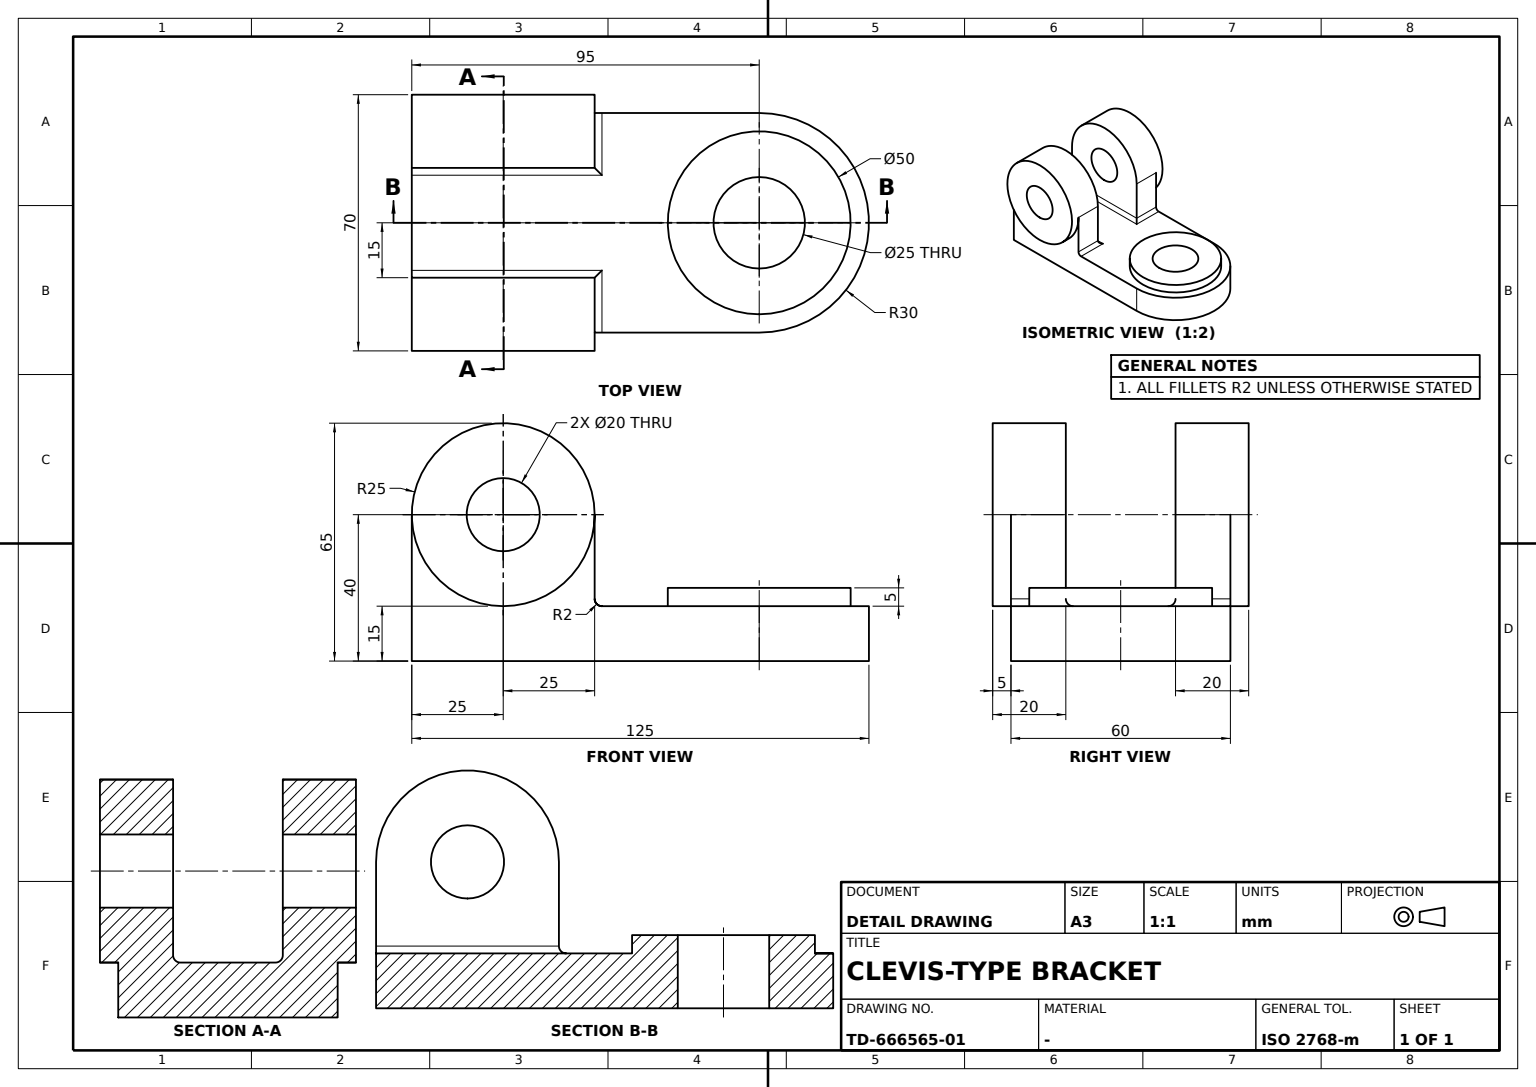
ISO-10303-21;
HEADER;
FILE_DESCRIPTION((''),'2;1');
FILE_NAME('','',(''),(''),'','','');
FILE_SCHEMA(('AUTOMOTIVE_DESIGN'));
ENDSEC;
DATA;
#1=APPLICATION_CONTEXT('');
#2=PRODUCT_CONTEXT('',#1,'mechanical');
#3=PRODUCT('','','',(#2));
#4=PRODUCT_DEFINITION_FORMATION('','',#3);
#5=PRODUCT_DEFINITION_CONTEXT('',#1,'design');
#6=PRODUCT_DEFINITION('','',#4,#5);
#7=PRODUCT_DEFINITION_SHAPE('','',#6);
#8=(LENGTH_UNIT()NAMED_UNIT(*)SI_UNIT(.MILLI.,.METRE.));
#9=(NAMED_UNIT(*)PLANE_ANGLE_UNIT()SI_UNIT($,.RADIAN.));
#10=(NAMED_UNIT(*)SI_UNIT($,.STERADIAN.)SOLID_ANGLE_UNIT());
#11=UNCERTAINTY_MEASURE_WITH_UNIT(LENGTH_MEASURE(0.005),#8,'distance_accuracy_value','');
#12=(GEOMETRIC_REPRESENTATION_CONTEXT(3)GLOBAL_UNCERTAINTY_ASSIGNED_CONTEXT((#11))GLOBAL_UNIT_ASSIGNED_CONTEXT((#8,#9,#10))REPRESENTATION_CONTEXT('',''));
#13=CARTESIAN_POINT('',(15.,-95.,40.));
#14=VERTEX_POINT('',#13);
#15=CARTESIAN_POINT('',(15.,-95.,17.));
#16=VERTEX_POINT('',#15);
#17=CARTESIAN_POINT('',(15.,-95.,0.));
#18=DIRECTION('',(0.,0.,-1.));
#19=VECTOR('',#18,1000.);
#20=LINE('',#17,#19);
#21=EDGE_CURVE('',#14,#16,#20,.T.);
#22=ORIENTED_EDGE('',*,*,#21,.F.);
#23=CARTESIAN_POINT('',(15.,-45.,40.));
#24=VERTEX_POINT('',#23);
#25=CARTESIAN_POINT('',(15.,-70.,40.));
#26=DIRECTION('',(1.,0.,0.));
#27=AXIS2_PLACEMENT_3D('',#25,#26,#18);
#28=CIRCLE('',#27,25.);
#29=EDGE_CURVE('',#24,#14,#28,.T.);
#30=ORIENTED_EDGE('',*,*,#29,.F.);
#31=CARTESIAN_POINT('',(15.,-45.,17.));
#32=VERTEX_POINT('',#31);
#33=CARTESIAN_POINT('',(15.,-45.,15.));
#34=DIRECTION('',(0.,0.,1.));
#35=VECTOR('',#34,1000.);
#36=LINE('',#33,#35);
#37=EDGE_CURVE('',#32,#24,#36,.T.);
#38=ORIENTED_EDGE('',*,*,#37,.F.);
#39=CARTESIAN_POINT('',(15.,-32.5,17.));
#40=DIRECTION('',(0.,1.,0.));
#41=VECTOR('',#40,1000.);
#42=LINE('',#39,#41);
#43=EDGE_CURVE('',#16,#32,#42,.T.);
#44=ORIENTED_EDGE('',*,*,#43,.F.);
#45=EDGE_LOOP('',(#22,#30,#38,#44));
#46=FACE_BOUND('',#45,.T.);
#47=CARTESIAN_POINT('',(15.,-70.,30.));
#48=VERTEX_POINT('',#47);
#49=CIRCLE('',#27,10.);
#50=EDGE_CURVE('',#48,#48,#49,.F.);
#51=ORIENTED_EDGE('',*,*,#50,.F.);
#52=EDGE_LOOP('',(#51));
#53=FACE_BOUND('',#52,.T.);
#54=CARTESIAN_POINT('',(15.,0.,0.));
#55=AXIS2_PLACEMENT_3D('',#54,#26,#40);
#56=PLANE('',#55);
#57=ADVANCED_FACE('',(#46,#53),#56,.F.);
#58=CARTESIAN_POINT('',(35.,-70.,30.));
#59=VERTEX_POINT('',#58);
#60=CARTESIAN_POINT('',(35.,-70.,40.));
#61=AXIS2_PLACEMENT_3D('',#60,#26,#18);
#62=CIRCLE('',#61,10.);
#63=EDGE_CURVE('',#59,#59,#62,.T.);
#64=ORIENTED_EDGE('',*,*,#63,.T.);
#65=EDGE_LOOP('',(#64));
#66=FACE_BOUND('',#65,.T.);
#67=ORIENTED_EDGE('',*,*,#50,.T.);
#68=EDGE_LOOP('',(#67));
#69=FACE_BOUND('',#68,.T.);
#70=CARTESIAN_POINT('',(-34.9,-70.,40.));
#71=AXIS2_PLACEMENT_3D('',#70,#26,#40);
#72=CYLINDRICAL_SURFACE('',#71,10.);
#73=ADVANCED_FACE('',(#66,#69),#72,.F.);
#74=CARTESIAN_POINT('',(30.,-95.,0.));
#75=VERTEX_POINT('',#74);
#76=CARTESIAN_POINT('',(30.,-95.,40.));
#77=VERTEX_POINT('',#76);
#78=LINE('',#74,#35);
#79=EDGE_CURVE('',#75,#77,#78,.T.);
#80=ORIENTED_EDGE('',*,*,#79,.F.);
#81=CARTESIAN_POINT('',(30.,0.,0.));
#82=VERTEX_POINT('',#81);
#83=LINE('',#81,#41);
#84=EDGE_CURVE('',#75,#82,#83,.T.);
#85=ORIENTED_EDGE('',*,*,#84,.T.);
#86=CARTESIAN_POINT('',(30.,0.,15.));
#87=VERTEX_POINT('',#86);
#88=CARTESIAN_POINT('',(30.,0.,7.5));
#89=LINE('',#88,#35);
#90=EDGE_CURVE('',#82,#87,#89,.T.);
#91=ORIENTED_EDGE('',*,*,#90,.T.);
#92=CARTESIAN_POINT('',(30.,-43.,15.));
#93=VERTEX_POINT('',#92);
#94=LINE('',#86,#41);
#95=EDGE_CURVE('',#93,#87,#94,.T.);
#96=ORIENTED_EDGE('',*,*,#95,.F.);
#97=CARTESIAN_POINT('',(30.,-45.,17.));
#98=VERTEX_POINT('',#97);
#99=CARTESIAN_POINT('',(30.,-43.,17.));
#100=AXIS2_PLACEMENT_3D('',#99,#26,#18);
#101=CIRCLE('',#100,2.);
#102=EDGE_CURVE('',#98,#93,#101,.T.);
#103=ORIENTED_EDGE('',*,*,#102,.F.);
#104=CARTESIAN_POINT('',(30.,-45.,40.));
#105=VERTEX_POINT('',#104);
#106=CARTESIAN_POINT('',(30.,-45.,15.));
#107=LINE('',#106,#35);
#108=EDGE_CURVE('',#98,#105,#107,.T.);
#109=ORIENTED_EDGE('',*,*,#108,.T.);
#110=CARTESIAN_POINT('',(30.,-70.,40.));
#111=AXIS2_PLACEMENT_3D('',#110,#26,#18);
#112=CIRCLE('',#111,25.);
#113=EDGE_CURVE('',#77,#105,#112,.T.);
#114=ORIENTED_EDGE('',*,*,#113,.F.);
#115=EDGE_LOOP('',(#80,#85,#91,#96,#103,#109,#114));
#116=FACE_BOUND('',#115,.T.);
#117=AXIS2_PLACEMENT_3D('',#74,#26,#40);
#118=PLANE('',#117);
#119=ADVANCED_FACE('',(#116),#118,.T.);
#120=CARTESIAN_POINT('',(25.,0.,15.));
#121=VERTEX_POINT('',#120);
#122=CARTESIAN_POINT('',(0.,0.,15.));
#123=AXIS2_PLACEMENT_3D('',#122,#34,#26);
#124=CIRCLE('',#123,25.);
#125=EDGE_CURVE('',#121,#121,#124,.T.);
#126=ORIENTED_EDGE('',*,*,#125,.F.);
#127=EDGE_LOOP('',(#126));
#128=FACE_BOUND('',#127,.T.);
#129=CARTESIAN_POINT('',(13.,-95.,15.));
#130=VERTEX_POINT('',#129);
#131=CARTESIAN_POINT('',(13.,-43.,15.));
#132=VERTEX_POINT('',#131);
#133=CARTESIAN_POINT('',(13.,-32.5,15.));
#134=LINE('',#133,#41);
#135=EDGE_CURVE('',#130,#132,#134,.T.);
#136=ORIENTED_EDGE('',*,*,#135,.T.);
#137=CARTESIAN_POINT('',(0.,-43.,15.));
#138=DIRECTION('',(-1.,0.,0.));
#139=VECTOR('',#138,1000.);
#140=LINE('',#137,#139);
#141=EDGE_CURVE('',#93,#132,#140,.T.);
#142=ORIENTED_EDGE('',*,*,#141,.F.);
#143=ORIENTED_EDGE('',*,*,#95,.T.);
#144=CARTESIAN_POINT('',(-30.,0.,15.));
#145=VERTEX_POINT('',#144);
#146=CIRCLE('',#123,30.);
#147=EDGE_CURVE('',#87,#145,#146,.T.);
#148=ORIENTED_EDGE('',*,*,#147,.T.);
#149=CARTESIAN_POINT('',(-30.,-43.,15.));
#150=VERTEX_POINT('',#149);
#151=DIRECTION('',(0.,-1.,0.));
#152=VECTOR('',#151,1000.);
#153=LINE('',#144,#152);
#154=EDGE_CURVE('',#145,#150,#153,.T.);
#155=ORIENTED_EDGE('',*,*,#154,.T.);
#156=CARTESIAN_POINT('',(-13.,-43.,15.));
#157=VERTEX_POINT('',#156);
#158=EDGE_CURVE('',#157,#150,#140,.T.);
#159=ORIENTED_EDGE('',*,*,#158,.F.);
#160=CARTESIAN_POINT('',(-13.,-95.,15.));
#161=VERTEX_POINT('',#160);
#162=CARTESIAN_POINT('',(-13.,-32.5,15.));
#163=LINE('',#162,#41);
#164=EDGE_CURVE('',#161,#157,#163,.T.);
#165=ORIENTED_EDGE('',*,*,#164,.F.);
#166=CARTESIAN_POINT('',(0.,-95.,15.));
#167=VECTOR('',#26,1000.);
#168=LINE('',#166,#167);
#169=EDGE_CURVE('',#161,#130,#168,.T.);
#170=ORIENTED_EDGE('',*,*,#169,.T.);
#171=EDGE_LOOP('',(#136,#142,#143,#148,#155,#159,#165,#170));
#172=FACE_BOUND('',#171,.T.);
#173=PLANE('',#123);
#174=ADVANCED_FACE('',(#128,#172),#173,.T.);
#175=CARTESIAN_POINT('',(32.5,-45.,40.));
#176=LINE('',#175,#167);
#177=EDGE_CURVE('',#105,#24,#176,.F.);
#178=ORIENTED_EDGE('',*,*,#177,.F.);
#179=ORIENTED_EDGE('',*,*,#108,.F.);
#180=CARTESIAN_POINT('',(0.,-45.,17.));
#181=LINE('',#180,#139);
#182=EDGE_CURVE('',#98,#32,#181,.T.);
#183=ORIENTED_EDGE('',*,*,#182,.T.);
#184=ORIENTED_EDGE('',*,*,#37,.T.);
#185=EDGE_LOOP('',(#178,#179,#183,#184));
#186=FACE_BOUND('',#185,.T.);
#187=AXIS2_PLACEMENT_3D('',#106,#151,#34);
#188=PLANE('',#187);
#189=ADVANCED_FACE('',(#186),#188,.F.);
#190=CARTESIAN_POINT('',(25.,0.,20.));
#191=VERTEX_POINT('',#190);
#192=CARTESIAN_POINT('',(0.,0.,20.));
#193=AXIS2_PLACEMENT_3D('',#192,#34,#26);
#194=CIRCLE('',#193,25.);
#195=EDGE_CURVE('',#191,#191,#194,.T.);
#196=ORIENTED_EDGE('',*,*,#195,.T.);
#197=EDGE_LOOP('',(#196));
#198=FACE_BOUND('',#197,.T.);
#199=CARTESIAN_POINT('',(12.5,0.,20.));
#200=VERTEX_POINT('',#199);
#201=CIRCLE('',#193,12.5);
#202=EDGE_CURVE('',#200,#200,#201,.T.);
#203=ORIENTED_EDGE('',*,*,#202,.F.);
#204=EDGE_LOOP('',(#203));
#205=FACE_BOUND('',#204,.T.);
#206=PLANE('',#193);
#207=ADVANCED_FACE('',(#198,#205),#206,.T.);
#208=CARTESIAN_POINT('',(-15.,-45.,17.));
#209=VERTEX_POINT('',#208);
#210=CARTESIAN_POINT('',(-30.,-45.,17.));
#211=VERTEX_POINT('',#210);
#212=EDGE_CURVE('',#209,#211,#181,.T.);
#213=ORIENTED_EDGE('',*,*,#212,.T.);
#214=CARTESIAN_POINT('',(-30.,-45.,40.));
#215=VERTEX_POINT('',#214);
#216=CARTESIAN_POINT('',(-30.,-45.,0.));
#217=LINE('',#216,#35);
#218=EDGE_CURVE('',#211,#215,#217,.T.);
#219=ORIENTED_EDGE('',*,*,#218,.T.);
#220=CARTESIAN_POINT('',(-15.,-45.,40.));
#221=VERTEX_POINT('',#220);
#222=EDGE_CURVE('',#215,#221,#176,.T.);
#223=ORIENTED_EDGE('',*,*,#222,.T.);
#224=CARTESIAN_POINT('',(-15.,-45.,15.));
#225=LINE('',#224,#35);
#226=EDGE_CURVE('',#209,#221,#225,.T.);
#227=ORIENTED_EDGE('',*,*,#226,.F.);
#228=EDGE_LOOP('',(#213,#219,#223,#227));
#229=FACE_BOUND('',#228,.T.);
#230=ADVANCED_FACE('',(#229),#188,.F.);
#231=CARTESIAN_POINT('',(-15.,-95.,17.));
#232=VERTEX_POINT('',#231);
#233=CARTESIAN_POINT('',(-15.,-32.5,17.));
#234=LINE('',#233,#41);
#235=EDGE_CURVE('',#232,#209,#234,.T.);
#236=ORIENTED_EDGE('',*,*,#235,.T.);
#237=ORIENTED_EDGE('',*,*,#226,.T.);
#238=CARTESIAN_POINT('',(-15.,-95.,40.));
#239=VERTEX_POINT('',#238);
#240=CARTESIAN_POINT('',(-15.,-70.,40.));
#241=AXIS2_PLACEMENT_3D('',#240,#26,#18);
#242=CIRCLE('',#241,25.);
#243=EDGE_CURVE('',#221,#239,#242,.T.);
#244=ORIENTED_EDGE('',*,*,#243,.T.);
#245=CARTESIAN_POINT('',(-15.,-95.,0.));
#246=LINE('',#245,#19);
#247=EDGE_CURVE('',#239,#232,#246,.T.);
#248=ORIENTED_EDGE('',*,*,#247,.T.);
#249=EDGE_LOOP('',(#236,#237,#244,#248));
#250=FACE_BOUND('',#249,.T.);
#251=CARTESIAN_POINT('',(-15.,-70.,30.));
#252=VERTEX_POINT('',#251);
#253=CIRCLE('',#241,10.);
#254=EDGE_CURVE('',#252,#252,#253,.T.);
#255=ORIENTED_EDGE('',*,*,#254,.F.);
#256=EDGE_LOOP('',(#255));
#257=FACE_BOUND('',#256,.T.);
#258=CARTESIAN_POINT('',(-15.,0.,0.));
#259=AXIS2_PLACEMENT_3D('',#258,#26,#40);
#260=PLANE('',#259);
#261=ADVANCED_FACE('',(#250,#257),#260,.T.);
#262=CARTESIAN_POINT('',(-30.,0.,0.));
#263=VERTEX_POINT('',#262);
#264=CARTESIAN_POINT('',(-30.,0.,7.5));
#265=LINE('',#264,#35);
#266=EDGE_CURVE('',#263,#145,#265,.T.);
#267=ORIENTED_EDGE('',*,*,#266,.T.);
#268=ORIENTED_EDGE('',*,*,#147,.F.);
#269=ORIENTED_EDGE('',*,*,#90,.F.);
#270=CARTESIAN_POINT('',(0.,0.,0.));
#271=AXIS2_PLACEMENT_3D('',#270,#34,#26);
#272=CIRCLE('',#271,30.);
#273=EDGE_CURVE('',#82,#263,#272,.T.);
#274=ORIENTED_EDGE('',*,*,#273,.T.);
#275=EDGE_LOOP('',(#267,#268,#269,#274));
#276=FACE_BOUND('',#275,.T.);
#277=CARTESIAN_POINT('',(0.,0.,7.5));
#278=AXIS2_PLACEMENT_3D('',#277,#34,#26);
#279=CYLINDRICAL_SURFACE('',#278,30.);
#280=ADVANCED_FACE('',(#276),#279,.T.);
#281=ORIENTED_EDGE('',*,*,#63,.F.);
#282=EDGE_LOOP('',(#281));
#283=FACE_BOUND('',#282,.T.);
#284=CARTESIAN_POINT('',(35.,-70.,15.));
#285=VERTEX_POINT('',#284);
#286=CIRCLE('',#61,25.);
#287=EDGE_CURVE('',#285,#285,#286,.T.);
#288=ORIENTED_EDGE('',*,*,#287,.T.);
#289=EDGE_LOOP('',(#288));
#290=FACE_BOUND('',#289,.T.);
#291=CARTESIAN_POINT('',(35.,0.,0.));
#292=AXIS2_PLACEMENT_3D('',#291,#26,#40);
#293=PLANE('',#292);
#294=ADVANCED_FACE('',(#283,#290),#293,.T.);
#295=CARTESIAN_POINT('',(-35.,-70.,50.));
#296=VERTEX_POINT('',#295);
#297=CARTESIAN_POINT('',(-35.,-70.,40.));
#298=AXIS2_PLACEMENT_3D('',#297,#138,#34);
#299=CIRCLE('',#298,10.);
#300=EDGE_CURVE('',#296,#296,#299,.T.);
#301=ORIENTED_EDGE('',*,*,#300,.T.);
#302=EDGE_LOOP('',(#301));
#303=FACE_BOUND('',#302,.T.);
#304=ORIENTED_EDGE('',*,*,#254,.T.);
#305=EDGE_LOOP('',(#304));
#306=FACE_BOUND('',#305,.T.);
#307=ADVANCED_FACE('',(#303,#306),#72,.F.);
#308=ORIENTED_EDGE('',*,*,#195,.F.);
#309=EDGE_LOOP('',(#308));
#310=FACE_BOUND('',#309,.T.);
#311=ORIENTED_EDGE('',*,*,#125,.T.);
#312=EDGE_LOOP('',(#311));
#313=FACE_BOUND('',#312,.T.);
#314=CARTESIAN_POINT('',(0.,0.,17.5));
#315=AXIS2_PLACEMENT_3D('',#314,#34,#26);
#316=CYLINDRICAL_SURFACE('',#315,25.);
#317=ADVANCED_FACE('',(#310,#313),#316,.T.);
#318=CARTESIAN_POINT('',(-30.,-95.,0.));
#319=VERTEX_POINT('',#318);
#320=CARTESIAN_POINT('',(-30.,-95.,40.));
#321=VERTEX_POINT('',#320);
#322=LINE('',#318,#35);
#323=EDGE_CURVE('',#319,#321,#322,.T.);
#324=ORIENTED_EDGE('',*,*,#323,.T.);
#325=CARTESIAN_POINT('',(-30.,-70.,40.));
#326=AXIS2_PLACEMENT_3D('',#325,#138,#34);
#327=CIRCLE('',#326,25.);
#328=EDGE_CURVE('',#215,#321,#327,.T.);
#329=ORIENTED_EDGE('',*,*,#328,.F.);
#330=ORIENTED_EDGE('',*,*,#218,.F.);
#331=CARTESIAN_POINT('',(-30.,-43.,17.));
#332=AXIS2_PLACEMENT_3D('',#331,#138,#34);
#333=CIRCLE('',#332,2.);
#334=EDGE_CURVE('',#150,#211,#333,.T.);
#335=ORIENTED_EDGE('',*,*,#334,.F.);
#336=ORIENTED_EDGE('',*,*,#154,.F.);
#337=ORIENTED_EDGE('',*,*,#266,.F.);
#338=LINE('',#262,#152);
#339=EDGE_CURVE('',#263,#319,#338,.T.);
#340=ORIENTED_EDGE('',*,*,#339,.T.);
#341=EDGE_LOOP('',(#324,#329,#330,#335,#336,#337,#340));
#342=FACE_BOUND('',#341,.T.);
#343=AXIS2_PLACEMENT_3D('',#262,#138,#151);
#344=PLANE('',#343);
#345=ADVANCED_FACE('',(#342),#344,.T.);
#346=ORIENTED_EDGE('',*,*,#43,.T.);
#347=CARTESIAN_POINT('',(13.,-43.,17.));
#348=DIRECTION('',(0.707106781,0.707106781,0.));
#349=DIRECTION('',(-0.707106781,0.707106781,0.));
#350=AXIS2_PLACEMENT_3D('',#347,#348,#349);
#351=ELLIPSE('',#350,2.828427,2.);
#352=EDGE_CURVE('',#32,#132,#351,.T.);
#353=ORIENTED_EDGE('',*,*,#352,.T.);
#354=ORIENTED_EDGE('',*,*,#135,.F.);
#355=CARTESIAN_POINT('',(13.,-95.,17.));
#356=AXIS2_PLACEMENT_3D('',#355,#151,#18);
#357=CIRCLE('',#356,2.);
#358=EDGE_CURVE('',#130,#16,#357,.T.);
#359=ORIENTED_EDGE('',*,*,#358,.T.);
#360=EDGE_LOOP('',(#346,#353,#354,#359));
#361=FACE_BOUND('',#360,.T.);
#362=CARTESIAN_POINT('',(13.,-32.5,17.));
#363=AXIS2_PLACEMENT_3D('',#362,#40,#26);
#364=CYLINDRICAL_SURFACE('',#363,2.);
#365=ADVANCED_FACE('',(#361),#364,.F.);
#366=CARTESIAN_POINT('',(32.5,-95.,40.));
#367=LINE('',#366,#167);
#368=EDGE_CURVE('',#77,#14,#367,.F.);
#369=ORIENTED_EDGE('',*,*,#368,.T.);
#370=ORIENTED_EDGE('',*,*,#21,.T.);
#371=ORIENTED_EDGE('',*,*,#358,.F.);
#372=ORIENTED_EDGE('',*,*,#169,.F.);
#373=CARTESIAN_POINT('',(-13.,-95.,17.));
#374=AXIS2_PLACEMENT_3D('',#373,#151,#18);
#375=CIRCLE('',#374,2.);
#376=EDGE_CURVE('',#232,#161,#375,.T.);
#377=ORIENTED_EDGE('',*,*,#376,.F.);
#378=ORIENTED_EDGE('',*,*,#247,.F.);
#379=EDGE_CURVE('',#321,#239,#367,.T.);
#380=ORIENTED_EDGE('',*,*,#379,.F.);
#381=ORIENTED_EDGE('',*,*,#323,.F.);
#382=CARTESIAN_POINT('',(0.,-95.,0.));
#383=LINE('',#382,#167);
#384=EDGE_CURVE('',#319,#75,#383,.T.);
#385=ORIENTED_EDGE('',*,*,#384,.T.);
#386=ORIENTED_EDGE('',*,*,#79,.T.);
#387=EDGE_LOOP('',(#369,#370,#371,#372,#377,#378,#380,#381,#385,#386));
#388=FACE_BOUND('',#387,.T.);
#389=AXIS2_PLACEMENT_3D('',#318,#151,#26);
#390=PLANE('',#389);
#391=ADVANCED_FACE('',(#388),#390,.T.);
#392=ORIENTED_EDGE('',*,*,#212,.F.);
#393=CARTESIAN_POINT('',(-13.,-43.,17.));
#394=DIRECTION('',(-0.707106781,-0.707106781,0.));
#395=AXIS2_PLACEMENT_3D('',#393,#349,#394);
#396=ELLIPSE('',#395,2.828427,2.);
#397=EDGE_CURVE('',#209,#157,#396,.F.);
#398=ORIENTED_EDGE('',*,*,#397,.T.);
#399=ORIENTED_EDGE('',*,*,#158,.T.);
#400=ORIENTED_EDGE('',*,*,#334,.T.);
#401=EDGE_LOOP('',(#392,#398,#399,#400));
#402=FACE_BOUND('',#401,.T.);
#403=CARTESIAN_POINT('',(0.,-43.,17.));
#404=AXIS2_PLACEMENT_3D('',#403,#138,#151);
#405=CYLINDRICAL_SURFACE('',#404,2.);
#406=ADVANCED_FACE('',(#402),#405,.F.);
#407=ORIENTED_EDGE('',*,*,#102,.T.);
#408=ORIENTED_EDGE('',*,*,#141,.T.);
#409=ORIENTED_EDGE('',*,*,#352,.F.);
#410=ORIENTED_EDGE('',*,*,#182,.F.);
#411=EDGE_LOOP('',(#407,#408,#409,#410));
#412=FACE_BOUND('',#411,.T.);
#413=ADVANCED_FACE('',(#412),#405,.F.);
#414=CARTESIAN_POINT('',(-35.,-70.,65.));
#415=VERTEX_POINT('',#414);
#416=CIRCLE('',#298,25.);
#417=EDGE_CURVE('',#415,#415,#416,.T.);
#418=ORIENTED_EDGE('',*,*,#417,.F.);
#419=EDGE_LOOP('',(#418));
#420=FACE_BOUND('',#419,.T.);
#421=ORIENTED_EDGE('',*,*,#328,.T.);
#422=ORIENTED_EDGE('',*,*,#379,.T.);
#423=ORIENTED_EDGE('',*,*,#243,.F.);
#424=ORIENTED_EDGE('',*,*,#222,.F.);
#425=EDGE_LOOP('',(#421,#422,#423,#424));
#426=FACE_BOUND('',#425,.T.);
#427=CARTESIAN_POINT('',(32.5,-70.,40.));
#428=AXIS2_PLACEMENT_3D('',#427,#26,#40);
#429=CYLINDRICAL_SURFACE('',#428,25.);
#430=ADVANCED_FACE('',(#420,#426),#429,.T.);
#431=ORIENTED_EDGE('',*,*,#417,.T.);
#432=EDGE_LOOP('',(#431));
#433=FACE_BOUND('',#432,.T.);
#434=ORIENTED_EDGE('',*,*,#300,.F.);
#435=EDGE_LOOP('',(#434));
#436=FACE_BOUND('',#435,.T.);
#437=CARTESIAN_POINT('',(-35.,0.,0.));
#438=AXIS2_PLACEMENT_3D('',#437,#138,#151);
#439=PLANE('',#438);
#440=ADVANCED_FACE('',(#433,#436),#439,.T.);
#441=ORIENTED_EDGE('',*,*,#235,.F.);
#442=ORIENTED_EDGE('',*,*,#376,.T.);
#443=ORIENTED_EDGE('',*,*,#164,.T.);
#444=ORIENTED_EDGE('',*,*,#397,.F.);
#445=EDGE_LOOP('',(#441,#442,#443,#444));
#446=FACE_BOUND('',#445,.T.);
#447=CARTESIAN_POINT('',(-13.,-32.5,17.));
#448=AXIS2_PLACEMENT_3D('',#447,#40,#138);
#449=CYLINDRICAL_SURFACE('',#448,2.);
#450=ADVANCED_FACE('',(#446),#449,.F.);
#451=ORIENTED_EDGE('',*,*,#287,.F.);
#452=EDGE_LOOP('',(#451));
#453=FACE_BOUND('',#452,.T.);
#454=ORIENTED_EDGE('',*,*,#368,.F.);
#455=ORIENTED_EDGE('',*,*,#113,.T.);
#456=ORIENTED_EDGE('',*,*,#177,.T.);
#457=ORIENTED_EDGE('',*,*,#29,.T.);
#458=EDGE_LOOP('',(#454,#455,#456,#457));
#459=FACE_BOUND('',#458,.T.);
#460=ADVANCED_FACE('',(#453,#459),#429,.T.);
#461=CARTESIAN_POINT('',(12.5,0.,0.));
#462=VERTEX_POINT('',#461);
#463=CIRCLE('',#271,12.5);
#464=EDGE_CURVE('',#462,#462,#463,.F.);
#465=ORIENTED_EDGE('',*,*,#464,.T.);
#466=EDGE_LOOP('',(#465));
#467=FACE_BOUND('',#466,.T.);
#468=ORIENTED_EDGE('',*,*,#202,.T.);
#469=EDGE_LOOP('',(#468));
#470=FACE_BOUND('',#469,.T.);
#471=CARTESIAN_POINT('',(0.,0.,19.9));
#472=AXIS2_PLACEMENT_3D('',#471,#18,#26);
#473=CYLINDRICAL_SURFACE('',#472,12.5);
#474=ADVANCED_FACE('',(#467,#470),#473,.F.);
#475=ORIENTED_EDGE('',*,*,#464,.F.);
#476=EDGE_LOOP('',(#475));
#477=FACE_BOUND('',#476,.T.);
#478=ORIENTED_EDGE('',*,*,#384,.F.);
#479=ORIENTED_EDGE('',*,*,#339,.F.);
#480=ORIENTED_EDGE('',*,*,#273,.F.);
#481=ORIENTED_EDGE('',*,*,#84,.F.);
#482=EDGE_LOOP('',(#478,#479,#480,#481));
#483=FACE_BOUND('',#482,.T.);
#484=PLANE('',#271);
#485=ADVANCED_FACE('',(#477,#483),#484,.F.);
#486=CLOSED_SHELL('',(#57,#73,#119,#174,#189,#207,#230,#261,#280,#294,#307,#317,#345,#365,#391,#406,#413,#430,#440,#450,#460,#474,#485));
#487=MANIFOLD_SOLID_BREP('',#486);
#488=ADVANCED_BREP_SHAPE_REPRESENTATION('',(#487),#12);
#489=SHAPE_DEFINITION_REPRESENTATION(#7,#488);
ENDSEC;
END-ISO-10303-21;
